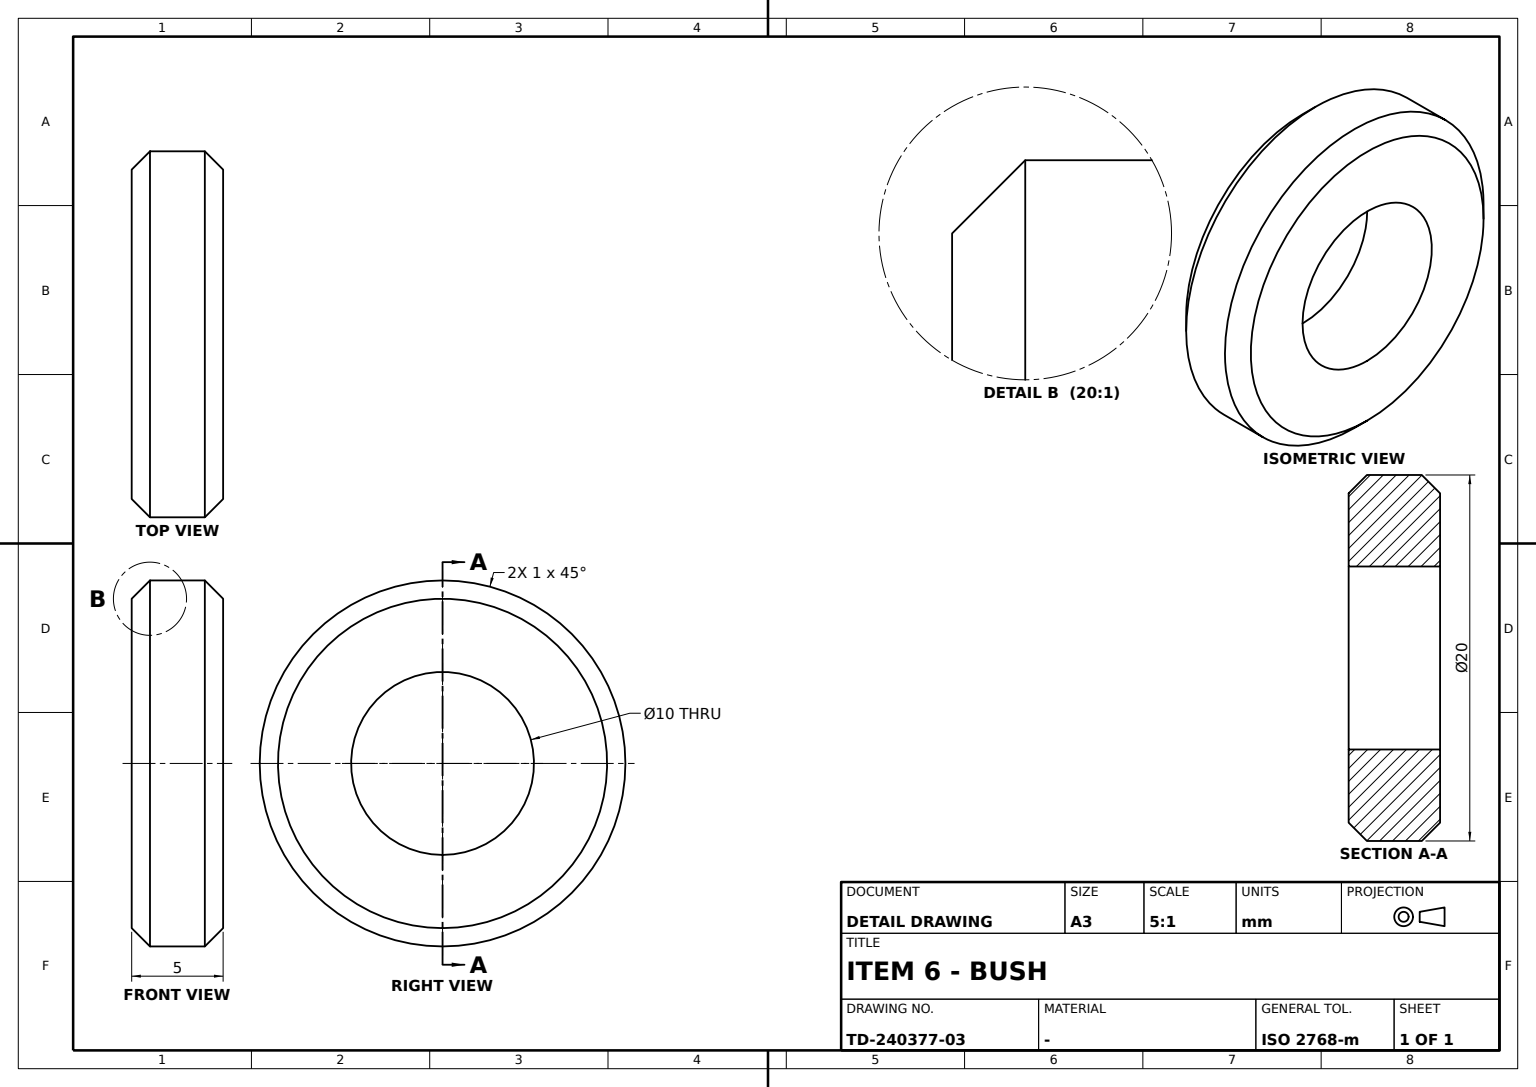
ISO-10303-21;
HEADER;
FILE_DESCRIPTION((''),'2;1');
FILE_NAME('','',(''),(''),'','','');
FILE_SCHEMA(('AUTOMOTIVE_DESIGN'));
ENDSEC;
DATA;
#1=APPLICATION_CONTEXT('');
#2=PRODUCT_CONTEXT('',#1,'mechanical');
#3=PRODUCT('','','',(#2));
#4=PRODUCT_DEFINITION_FORMATION('','',#3);
#5=PRODUCT_DEFINITION_CONTEXT('',#1,'design');
#6=PRODUCT_DEFINITION('','',#4,#5);
#7=PRODUCT_DEFINITION_SHAPE('','',#6);
#8=(LENGTH_UNIT()NAMED_UNIT(*)SI_UNIT(.MILLI.,.METRE.));
#9=(NAMED_UNIT(*)PLANE_ANGLE_UNIT()SI_UNIT($,.RADIAN.));
#10=(NAMED_UNIT(*)SI_UNIT($,.STERADIAN.)SOLID_ANGLE_UNIT());
#11=UNCERTAINTY_MEASURE_WITH_UNIT(LENGTH_MEASURE(0.005),#8,'distance_accuracy_value','');
#12=(GEOMETRIC_REPRESENTATION_CONTEXT(3)GLOBAL_UNCERTAINTY_ASSIGNED_CONTEXT((#11))GLOBAL_UNIT_ASSIGNED_CONTEXT((#8,#9,#10))REPRESENTATION_CONTEXT('',''));
#13=CARTESIAN_POINT('',(-2.5,0.,-9.));
#14=VERTEX_POINT('',#13);
#15=CARTESIAN_POINT('',(-2.5,0.,0.));
#16=DIRECTION('',(1.,0.,0.));
#17=DIRECTION('',(0.,0.,-1.));
#18=AXIS2_PLACEMENT_3D('',#15,#16,#17);
#19=CIRCLE('',#18,9.);
#20=EDGE_CURVE('',#14,#14,#19,.T.);
#21=ORIENTED_EDGE('',*,*,#20,.F.);
#22=EDGE_LOOP('',(#21));
#23=FACE_BOUND('',#22,.T.);
#24=CARTESIAN_POINT('',(-2.5,0.,-5.));
#25=VERTEX_POINT('',#24);
#26=CIRCLE('',#18,5.);
#27=EDGE_CURVE('',#25,#25,#26,.T.);
#28=ORIENTED_EDGE('',*,*,#27,.T.);
#29=EDGE_LOOP('',(#28));
#30=FACE_BOUND('',#29,.T.);
#31=DIRECTION('',(0.,1.,0.));
#32=AXIS2_PLACEMENT_3D('',#15,#16,#31);
#33=PLANE('',#32);
#34=ADVANCED_FACE('',(#23,#30),#33,.F.);
#35=CARTESIAN_POINT('',(2.5,0.,-5.));
#36=VERTEX_POINT('',#35);
#37=CARTESIAN_POINT('',(2.5,0.,0.));
#38=AXIS2_PLACEMENT_3D('',#37,#16,#17);
#39=CIRCLE('',#38,5.);
#40=EDGE_CURVE('',#36,#36,#39,.T.);
#41=ORIENTED_EDGE('',*,*,#40,.T.);
#42=EDGE_LOOP('',(#41));
#43=FACE_BOUND('',#42,.T.);
#44=ORIENTED_EDGE('',*,*,#27,.F.);
#45=EDGE_LOOP('',(#44));
#46=FACE_BOUND('',#45,.T.);
#47=CARTESIAN_POINT('',(0.,0.,0.));
#48=AXIS2_PLACEMENT_3D('',#47,#16,#31);
#49=CYLINDRICAL_SURFACE('',#48,5.);
#50=ADVANCED_FACE('',(#43,#46),#49,.F.);
#51=CARTESIAN_POINT('',(1.5,-10.,0.));
#52=VERTEX_POINT('',#51);
#53=CARTESIAN_POINT('',(1.5,0.,0.));
#54=DIRECTION('',(-1.,0.,0.));
#55=DIRECTION('',(0.,-1.,0.));
#56=AXIS2_PLACEMENT_3D('',#53,#54,#55);
#57=CIRCLE('',#56,10.);
#58=EDGE_CURVE('',#52,#52,#57,.F.);
#59=ORIENTED_EDGE('',*,*,#58,.F.);
#60=EDGE_LOOP('',(#59));
#61=FACE_BOUND('',#60,.T.);
#62=CARTESIAN_POINT('',(-1.5,0.,-10.));
#63=VERTEX_POINT('',#62);
#64=CARTESIAN_POINT('',(-1.5,0.,0.));
#65=AXIS2_PLACEMENT_3D('',#64,#16,#17);
#66=CIRCLE('',#65,10.);
#67=EDGE_CURVE('',#63,#63,#66,.T.);
#68=ORIENTED_EDGE('',*,*,#67,.T.);
#69=EDGE_LOOP('',(#68));
#70=FACE_BOUND('',#69,.T.);
#71=CYLINDRICAL_SURFACE('',#48,10.);
#72=ADVANCED_FACE('',(#61,#70),#71,.T.);
#73=ORIENTED_EDGE('',*,*,#20,.T.);
#74=EDGE_LOOP('',(#73));
#75=FACE_BOUND('',#74,.T.);
#76=ORIENTED_EDGE('',*,*,#67,.F.);
#77=EDGE_LOOP('',(#76));
#78=FACE_BOUND('',#77,.T.);
#79=CARTESIAN_POINT('',(-11.5,0.,0.));
#80=DIRECTION('',(0.,-0.959299053,0.282392149));
#81=AXIS2_PLACEMENT_3D('',#79,#16,#80);
#82=CONICAL_SURFACE('',#81,0.,0.785398163);
#83=ADVANCED_FACE('',(#75,#78),#82,.T.);
#84=ORIENTED_EDGE('',*,*,#40,.F.);
#85=EDGE_LOOP('',(#84));
#86=FACE_BOUND('',#85,.T.);
#87=CARTESIAN_POINT('',(2.5,0.,-9.));
#88=VERTEX_POINT('',#87);
#89=CIRCLE('',#38,9.);
#90=EDGE_CURVE('',#88,#88,#89,.T.);
#91=ORIENTED_EDGE('',*,*,#90,.T.);
#92=EDGE_LOOP('',(#91));
#93=FACE_BOUND('',#92,.T.);
#94=AXIS2_PLACEMENT_3D('',#37,#16,#31);
#95=PLANE('',#94);
#96=ADVANCED_FACE('',(#86,#93),#95,.T.);
#97=ORIENTED_EDGE('',*,*,#58,.T.);
#98=EDGE_LOOP('',(#97));
#99=FACE_BOUND('',#98,.T.);
#100=ORIENTED_EDGE('',*,*,#90,.F.);
#101=EDGE_LOOP('',(#100));
#102=FACE_BOUND('',#101,.T.);
#103=CARTESIAN_POINT('',(11.5,0.,0.));
#104=DIRECTION('',(0.,0.959299053,-0.282392149));
#105=AXIS2_PLACEMENT_3D('',#103,#54,#104);
#106=CONICAL_SURFACE('',#105,0.,0.785398163);
#107=ADVANCED_FACE('',(#99,#102),#106,.T.);
#108=CLOSED_SHELL('',(#34,#50,#72,#83,#96,#107));
#109=MANIFOLD_SOLID_BREP('',#108);
#110=ADVANCED_BREP_SHAPE_REPRESENTATION('',(#109),#12);
#111=SHAPE_DEFINITION_REPRESENTATION(#7,#110);
ENDSEC;
END-ISO-10303-21;
